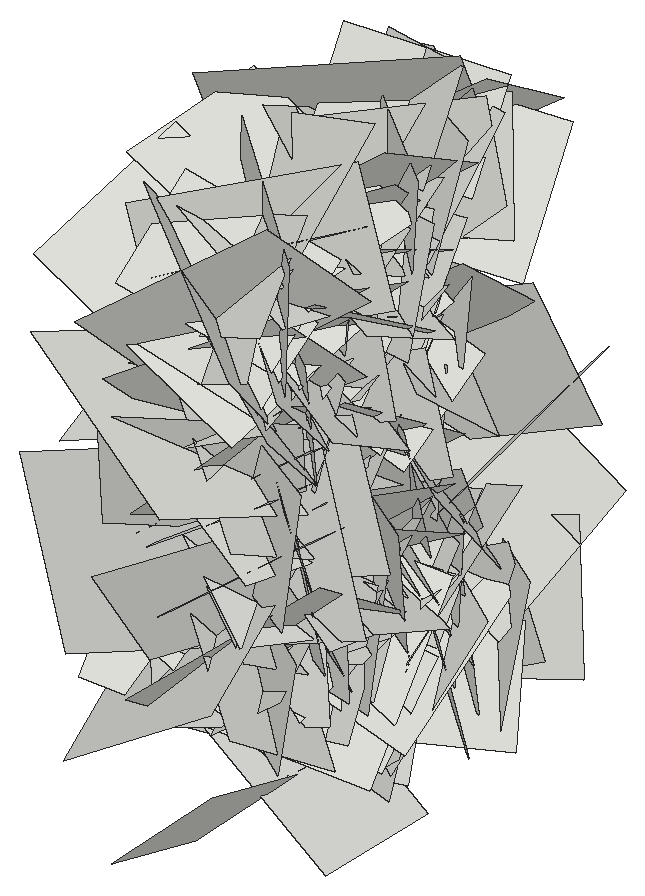
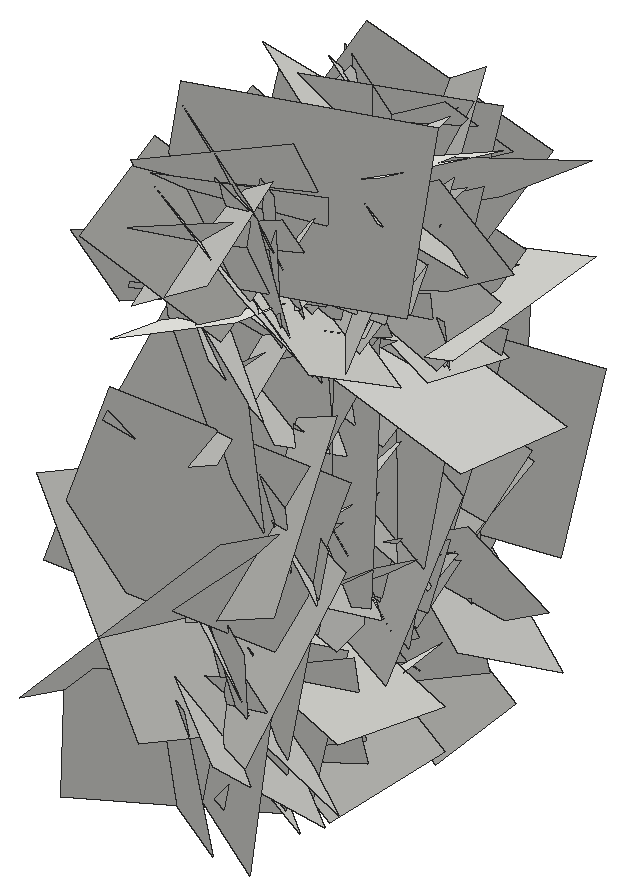
# SketchUp Ruby script. Lengths in inches.
U = 1.inch
M = Sketchup.active_model
def pt(a) = Geom::Point3d.new(a.map { |v| v * U })
def face(e, loops, mat)
  f = e.add_face(loops[0].map { |a| pt(a) })
  loops[1..].each { |l| e.add_face(l.map { |a| pt(a) }).erase! }
  f.material = f.back_material = mat if mat
  f
end
# faces: each face lists its corners as indices into pts; further lists are holes
def faces(e, pts, list, mat = nil) = list.each { |f| face(e, (f[0].is_a?(Array) ? f : [f]).map { |l| l.map { |i| pts[i] } }, mat) }
# xy, xz, yz: faces in a plane at the given z, y or x. An outline is a flat list of corners, or four numbers for a rectangle; further outlines are holes
def ring(l) = l.size == 4 ? [[l[0], l[1]], [l[2], l[1]], [l[2], l[3]], [l[0], l[3]]] : l.each_slice(2).to_a
def flat(e, list, mat, &to3) = list.each { |f| face(e, (f[0].is_a?(Array) ? f : [f]).map { |l| ring(l).map { |u, v| to3.(u, v) } }, mat) }
def xy(e, z, list, mat = nil) = flat(e, list, mat) { |x, y| [x, y, z] }
def xz(e, y, list, mat = nil) = flat(e, list, mat) { |x, z| [x, y, z] }
def yz(e, x, list, mat = nil) = flat(e, list, mat) { |y, z| [x, y, z] }
def lines(e, pts, list) = list.each { |a, b| e.add_line(pt(pts[a]), pt(pts[b])) }
# prism: a flat outline (further loops are holes) pulled along v
def prism(e, loops, v, mat = nil)
  f = face(e, loops, mat); d = Geom::Vector3d.new(v.map { |x| x * U })
  f.pushpull(f.normal.samedirection?(d) ? d.length : -d.length)
end
def box(e, o, s, mat = nil) = prism(e, [[o, [o[0] + s[0], o[1], o[2]], [o[0] + s[0], o[1] + s[1], o[2]], [o[0], o[1] + s[1], o[2]]]], [0, 0, s[2]], mat)
def at(x, y, z, deg = 0) = Geom::Transformation.translation(pt([x, y, z])) * Geom::Transformation.rotation(ORIGIN, Z_AXIS, deg.degrees)
def axes(o, x, y, z) = Geom::Transformation.new([*x, 0, *y, 0, *z, 0, *pt(o).to_a, 1])
def part(name) = M.definitions.add(name)
# library, detail: a bought-in or finely detailed component or shape, given as its bounding box
def library(name, o, s) = part(name).tap { |d| box(d.entities, o, s) }
def detail(e, o, s) = box(e.add_group.entities, o, s)
def put(e, d, t, mat = nil) = e.add_instance(d, t).tap { |i| i.material = mat if mat }
def group(e, t, mat = nil) = e.add_group.tap { |g| g.transformation = t; g.material = mat if mat }.entities
root = M.entities
c1 = part("Component\#6")
p = [[0.01,0,0],[0,3.24,4.54],[4.32,3.24,4.54],[4.33,0,0]]
faces(c1.entities,p,[[0,1,2,3]])
put(root,c1,axes([18.5,193.54,33.12],[-0.22081,1.30446,0.31828],[-0.37279,0.25784,-1.28691],[-1.3736,-0.27967,0.29809]))
put(root,c1,axes([18.5,195.625,24.52],[-0.22176,-0.47224,1.18941],[-0.10161,1.2076,0.46259],[-1.3527,-0.0133,-0.22974]))
put(root,c1,axes([18.5,200.57,23.13],[-0.2198,-0.69796,1.13548],[0.0671,1.14269,0.71395],[-1.41122,0.16304,-0.1429]))
put(root,c1,axes([18.5,199.97,41.09],[-0.2759,0.65189,-0.94787],[-0.07756,-0.97924,-0.65337],[-1.21695,-0.08538,0.25653]))
put(root,c1,axes([18.5,193.84,30.46],[-0.25587,-1.06575,0.3461],[-0.15582,0.3811,1.07099],[-1.17751,0.18115,-0.21693]))
put(root,c1,axes([18.5,194.52,25.48],[-0.11423,-0.20624,1.26777],[-0.06819,1.2715,0.20138],[-1.3598,-0.04643,-0.1166]))
put(root,c1,axes([18.5,189.88,26.35],[-0.12674,1.17916,0.69894],[0.07675,0.70605,-1.17877],[-1.45096,-0.06565,-0.1234]))
put(root,c1,axes([18.5,196.54,35.06],[-0.17609,-1.11494,-0.45613],[0.00034,-0.46049,1.12547],[-1.27691,0.15363,0.0632]))
put(root,c1,axes([18.5,199.72,26.12],[0.08735,-0.8928,-1.02237],[-0.07635,-1.02569,0.88989],[-1.43674,0.00023,-0.10945]))
put(root,c1,axes([18.5,196.35,30.1],[-0.25467,1.00338,0.64071],[0.12934,0.67094,-1.00496],[-1.25528,-0.13443,-0.23354]))
put(root,c1,axes([18.5,198.29,23.22],[-0.04433,-0.32511,1.32538],[0.126,1.3201,0.32757],[-1.44106,0.12543,-0.01213]))
put(root,c1,axes([18.5,200.75,21.625],[-0.14431,-0.01788,1.13958],[-0.06693,1.14604,0.01044],[-1.20625,-0.06145,-0.13692]))
put(root,c1,axes([18.5,197.21,31.46],[-0.04455,0.58157,-0.95839],[-0.2239,-0.94599,-0.56478],[-1.16701,0.1593,0.14494]))
put(root,c1,axes([18.5,198.24,37.08],[-0.15669,-0.99926,-0.19378],[-0.22295,-0.1616,0.99377],[-1.05566,0.18244,-0.18112]))
put(root,c1,axes([18.5,193.85,32.27],[-0.12737,1.17977,-0.33684],[0.1012,-0.32843,-1.18439],[-1.29659,-0.14153,-0.05935]))
put(root,c1,axes([18.5,196.04,25.17],[-0.02819,1.07686,0.22249],[-0.25409,0.21152,-1.05244],[-1.13755,-0.07393,0.22957]))
put(root,c1,axes([18.5,194.3,32.47],[0.23408,0.14056,-1.33491],[-0.22407,-1.33233,-0.17526],[-1.40507,0.23589,-0.19445]))
put(root,c1,axes([18.5,197.73,24.08],[-0.06299,0.80841,0.87356],[0.01823,0.87514,-0.8087],[-1.26151,-0.02772,-0.0553]))
put(root,c1,axes([18.5,195.34,33.06],[-0.01901,1.14103,-0.72029],[0.19621,-0.71146,-1.13165],[-1.41679,-0.11384,-0.14706]))
put(root,c1,axes([18.5,196.35,35.86],[-0.06555,0.97369,0.5362],[-0.0688,0.53295,-0.97527],[-1.17625,-0.08544,0.02716]))
put(root,c1,axes([18.5,198.78,35.93],[-0.06513,-0.64723,-0.92238],[-0.00055,-0.92374,0.64822],[-1.19442,0.03572,0.05]))
put(root,c1,axes([18.5,200.11,31.93],[-0.08158,0.26048,1.04137],[-0.05734,1.04178,-0.26458],[-1.13642,-0.07126,-0.06141]))
put(root,c1,axes([18.5,202.23,24.6],[0.19755,-1.2824,-0.48224],[0.04087,-0.48158,1.29554],[-1.4517,-0.18807,-0.02915]))
put(root,c1,axes([14.53,203.75,35.72],[-0.12855,-0.35471,-0.52952],[-0.05195,-0.53223,0.36775],[0.67359,-0.10874,-0.07269]))
put(root,c1,axes([18.5,192.77,37.47],[0.01566,0.85002,0.74451],[-0.07038,0.74394,-0.84805],[-1.19569,-0.03266,0.05967]))
put(root,c1,axes([18.5,197.22,25.56],[-0.17769,-0.12121,-0.94504],[-0.07151,-0.95564,0.13453],[-1.00742,0.08922,0.15714]))
put(root,c1,axes([18.5,195.04,27.27],[-0.2131,0.57774,0.71728],[-0.02179,0.73117,-0.59469],[-0.97604,-0.14247,-0.14333]))
put(root,c1,axes([18.5,201.66,25.46],[0.21728,-0.88431,0.94199],[-0.03627,0.94972,0.89901],[-1.36907,-0.16551,0.12568]))
put(root,c1,axes([18.5,202.95,33.21],[0.17447,0.42234,-1.07867],[-0.17991,-1.06896,-0.44444],[-1.21466,0.21899,-0.08911]))
put(root,c1,axes([18.5,199.05,27.98],[-0.08019,0.19915,0.92966],[-0.13728,0.92174,-0.20799],[-0.9984,-0.14274,-0.04607]))
put(root,c1,axes([18.5,197.83,24.35],[0.09568,0.96283,0.81475],[0.1112,0.80827,-0.9668],[-1.33234,0.1366,-0.02218]))
put(root,c1,axes([18.5,191.97,33.56],[-0.08688,0.89449,0.25558],[-0.12211,0.24484,-0.89383],[-0.97851,-0.10998,0.08885]))
put(root,c1,axes([18.5,196.22,30.25],[0.08073,-0.93811,0.99109],[0.27356,0.98462,0.91216],[-1.42044,0.13631,0.232]))
put(root,c1,axes([14.53,194.26,19.42],[-0.05867,-0.70774,0.13488],[-0.12622,0.14241,0.69835],[0.75321,-0.03127,0.12754]))
put(root,c1,axes([18.5,199.8,22.82],[0.00598,0.07204,1.08492],[0.02761,1.08461,-0.07215],[-1.15221,0.02636,0.0039]))
put(root,c1,axes([14.53,192.39,25.48],[-0.15082,-0.34829,0.66058],[-0.01541,0.67363,0.35204],[0.79143,-0.05326,0.13274]))
put(root,c1,axes([14.53,196.3,29.33],[-0.09147,0.43894,-0.4809],[0.05464,-0.47898,-0.44644],[0.688,0.09639,-0.02848]))
put(root,c1,axes([18.5,197.85,24.73],[0.35143,-0.52734,1.13432],[-0.18025,1.14359,0.58135],[-1.31365,-0.29799,0.22369]))
put(root,c1,axes([18.5,193.58,33.2],[-0.1306,0.22319,-0.86205],[-0.05382,-0.87061,-0.21815],[-0.94237,0.01879,0.13193]))
put(root,c1,axes([18.5,198.8,27.02],[0.0226,-0.2767,0.96977],[-0.06915,0.96758,0.27751],[-1.06674,-0.06859,0.00256]))
put(root,c1,axes([18.5,197.34,38.49],[-0.22162,0.66132,-0.53694],[0.02723,-0.54773,-0.68462],[-0.90256,-0.17891,0.1112]))
put(root,c1,axes([14.53,200.57,36.04],[-0.10099,0.61602,0.17436],[0.1325,0.19079,-0.60575],[0.66557,0.05549,0.14705]))
put(root,c1,axes([18.5,195.125,35.61],[-0.03117,0.92717,-0.40656],[0.02653,-0.40594,-0.92757],[-1.07281,-0.03698,-0.01113]))
put(root,c1,axes([14.53,198.68,37.125],[0.06347,0.58127,-0.24952],[-0.07215,-0.24326,-0.58302],[0.66662,-0.08167,-0.03935]))
put(root,c1,axes([14.53,193.25,29.42],[-0.0602,0.67546,-0.3863],[-0.10598,-0.39045,-0.66802],[0.81797,-0.00088,-0.11498]))
put(root,c1,axes([14.53,194.71,36.49],[-0.01491,0.71707,-0.22931],[-0.11795,-0.22881,-0.70868],[0.78925,-0.02064,-0.11024]))
put(root,c1,axes([18.5,198.67,35.61],[0.10111,0.59855,0.78971],[-0.15679,0.79307,-0.58323],[-1.03859,-0.06146,0.16492]))
put(root,c1,axes([18.5,206.72,25.52],[0.07134,-1.27871,-0.42932],[0.37284,-0.39835,1.24159],[-1.38032,-0.17369,0.31318]))
put(root,c1,axes([18.5,196.41,37.05],[-0.02372,0.78814,-0.36288],[-0.15491,-0.36124,-0.77556],[-0.90659,0.0411,0.14202]))
put(root,c1,axes([18.5,200.08,36.17],[-0.04967,-0.3024,-0.77978],[-0.15753,-0.76557,0.30582],[-0.87244,0.15545,-0.01082]))
put(root,c1,axes([14.53,194.0625,27.88],[-0.03826,-0.32146,0.75655],[-0.14724,0.74878,0.31153],[0.85881,0.11405,0.08712]))
put(root,c1,axes([14.53,192.62,23.41],[-0.0945,0.05137,0.75973],[0.00531,0.76494,-0.05113],[0.80713,0.00098,0.08928]))
put(root,c1,axes([14.53,194.1,30.97],[-0.07757,0.18705,0.69229],[0.05179,0.69557,-0.18277],[0.75837,-0.02837,0.08329]))
put(root,c1,axes([18.5,192.76,27.5],[0.21382,-0.08753,1.03604],[-0.20559,1.03367,0.1251],[-1.08277,-0.21355,0.18084]))
put(root,c1,axes([14.53,197.11,20.7],[-0.0234,0.20043,0.60552],[0.11848,0.59772,-0.19378],[0.66563,-0.09934,0.05578]))
put(root,c1,axes([18.5,194.12,36.42],[0.16155,0.92195,-0.51802],[-0.06641,-0.51458,-0.93426],[-1.119,0.16364,-0.01934]))
put(root,c1,axes([14.53,192.68,25.51],[0.10584,0.56729,0.32604],[-0.07365,0.33715,-0.56532],[0.68964,-0.05105,-0.11041]))
put(root,c1,axes([18.5,198.72,19.65],[0.06387,-1.04135,0.05905],[0.06023,0.06234,1.04135],[-1.10396,-0.05685,0.06023]))
put(root,c1,axes([18.5,194.92,22.54],[-0.07164,-0.895,0.57486],[0.24411,0.55005,0.88344],[-1.1008,0.18023,0.15849]))
put(root,c1,axes([18.5,200.17,25.9],[-0.12286,-0.34825,-0.84521],[0.12526,-0.85054,0.33424],[-0.96086,-0.06635,0.15165]))
put(root,c1,axes([14.53,196.5,26.6],[-0.00001,0.64808,0.59207],[-0.20568,0.57742,-0.63205],[0.90746,0.13088,-0.14325]))
put(root,c1,axes([18.5,195.45,23.05],[-0.08121,0.42866,0.62692],[-0.16296,0.6083,-0.43472],[-0.78836,-0.1699,0.02528]))
put(root,c1,axes([14.53,201.07,39.9375],[-0.03161,0.68058,-0.41337],[-0.06223,-0.41441,-0.67806],[0.84176,-0.00508,-0.06565]))
put(root,c1,axes([14.53,199.74,34.07],[0.11183,-0.60219,-0.2199],[-0.02555,-0.22643,0.6085],[0.67907,0.09065,0.0591]))
put(root,c1,axes([18.5,195.7,29.31],[0.12944,0.87645,-0.3909],[-0.13192,-0.37627,-0.88251],[-1.00866,0.16168,0.06525]))
put(root,c1,axes([18.5,195.4,26.27],[-0.15303,-0.80886,0.21466],[0.08059,0.20425,0.82078],[-0.8834,0.15875,0.0377]))
put(root,c1,axes([14.53,197.17,21.41],[-0.31691,0.51794,0.91951],[-0.05422,0.94746,-0.55031],[1.11735,0.19287,0.23409]))
put(root,c1,axes([18.5,204.82,25.65],[0.12938,-0.11687,-1.00907],[-0.02351,-1.01639,0.11504],[-1.07651,0.00815,-0.12379]))
put(root,c1,axes([14.53,192.15,39.48],[-0.21361,0.71392,-0.72381],[-0.12034,-0.74908,-0.70723],[1.07091,0.05823,-0.22384]))
put(root,c1,axes([18.5,200.1,34.99],[-0.01875,0.74709,-0.59948],[0.09315,-0.59579,-0.74508],[-1.01106,-0.06874,-0.05753]))
put(root,c1,axes([14.53,198.57,33.25],[-0.09717,0.14422,-0.89801],[-0.11089,-0.89824,-0.13357],[0.95769,-0.08937,-0.10658]))
put(root,c1,axes([18.5,201.91,26.14],[0.02369,0.31708,-0.9382],[0.09459,-0.93526,-0.31396],[-1.04548,-0.07743,-0.04967]))
put(root,c1,axes([18.5,195.16,37.28],[-0.08536,-0.54597,-0.55526],[-0.06407,-0.55215,0.55168],[-0.82294,0.09962,0.01464]))
put(root,c1,axes([14.53,196.95,39.61],[-0.06663,0.78722,-0.39485],[-0.0883,-0.3994,-0.78302],[0.92935,0.01849,-0.10271]))
put(root,c1,axes([14.53,194.17,31.15],[-0.1572,-0.65225,0.62778],[-0.00257,0.63643,0.66066],[0.9596,-0.10514,0.10461]))
put(root,c1,axes([18.5,197.53,26.62],[-0.11622,-0.11144,-0.6986],[-0.08861,-0.69994,0.12478],[-0.74462,0.10068,0.09418]))
put(root,c1,axes([18.5,195.33,34.42],[-0.12228,0.30682,0.85432],[0.19875,0.85067,-0.2802],[-0.94146,0.13973,-0.17012]))
put(root,c1,axes([14.53,195.89,35.57],[-0.03273,-0.74668,0.19464],[0.06894,0.19158,0.74527],[0.81502,-0.04619,-0.05522]))
put(root,c1,axes([14.53,192.38,31.46],[0.05244,0.73173,-0.11131],[0.01157,-0.11227,-0.73318],[0.78447,-0.04726,0.01825]))
put(root,c1,axes([18.5,198.41,25.5],[0.14641,-1.02966,0.26735],[0.10928,0.28128,1.03005],[-1.12233,-0.10694,0.13517]))
put(root,c1,axes([18.5,198.86,35.2],[0.14047,0.16017,0.87964],[-0.13868,0.88315,-0.1411],[-0.93754,-0.10664,0.15267]))
put(root,c1,axes([14.53,193.07,33.95],[0.05953,0.85388,-0.40475],[-0.24794,-0.38029,-0.83472],[0.97048,-0.14953,-0.18843]))
put(root,c1,axes([14.53,201.02,39.48],[-0.13577,0.09163,-0.9618],[-0.05798,-0.96935,-0.08506],[1.02248,-0.0428,-0.13253]))
put(root,c1,axes([14.53,192.92,34.17],[-0.15147,-0.1521,1.01718],[-0.1212,1.02293,0.1369],[1.08344,0.09316,0.15752]))
put(root,c1,axes([18.5,191.375,35.34],[-0.1473,0.40574,0.51918],[-0.07991,0.51733,-0.42447],[-0.69387,-0.14571,-0.06134]))
put(root,c1,axes([18.5,194.18,31.13],[0.04063,-0.16003,0.87853],[0.02386,0.87924,0.15917],[-0.94627,0.0153,0.04174]))
put(root,c1,axes([14.53,202.06,39.63],[-0.00244,-0.36914,-0.6705],[0.07457,-0.66776,0.36739],[0.80789,0.06052,-0.03594]))
put(root,c1,axes([18.5,201.02,32],[0.03236,-0.79816,-0.43551],[0.07074,-0.43262,0.79753],[-0.9612,-0.0587,0.04403]))
put(root,c1,axes([18.5,199.18,25.47],[-0.11604,-0.3767,0.6399],[0.02749,0.64448,0.38383],[-0.78661,0.07809,-0.08099]))
put(root,c1,axes([14.53,199.18,25.47],[0.11604,-0.3767,0.6399],[-0.02749,0.64448,0.38383],[0.78661,0.07809,-0.08099]))
put(root,c1,axes([14.53,201.02,32],[-0.03236,-0.79816,-0.43551],[-0.07074,-0.43262,0.79753],[0.9612,-0.0587,0.04403]))
put(root,c1,axes([18.5,202.06,39.63],[0.00244,-0.36914,-0.6705],[-0.07457,-0.66776,0.36739],[-0.80789,0.06052,-0.03594]))
put(root,c1,axes([14.53,194.18,31.13],[-0.04063,-0.16003,0.87853],[-0.02386,0.87924,0.15917],[0.94627,0.0153,0.04174]))
put(root,c1,axes([14.53,191.375,35.34],[0.1473,0.40574,0.51918],[0.07991,0.51733,-0.42447],[0.69387,-0.14571,-0.06134]))
put(root,c1,axes([18.5,192.92,34.17],[0.15147,-0.1521,1.01718],[0.1212,1.02293,0.1369],[-1.08344,0.09316,0.15752]))
put(root,c1,axes([18.5,201.02,39.48],[0.13577,0.09163,-0.9618],[0.05798,-0.96935,-0.08506],[-1.02248,-0.0428,-0.13253]))
put(root,c1,axes([18.5,193.07,33.95],[-0.05953,0.85388,-0.40475],[0.24794,-0.38029,-0.83472],[-0.97048,-0.14953,-0.18843]))
put(root,c1,axes([14.53,198.86,35.2],[-0.14047,0.16017,0.87964],[0.13868,0.88315,-0.1411],[0.93754,-0.10664,0.15267]))
put(root,c1,axes([14.53,198.41,25.5],[-0.14641,-1.02966,0.26735],[-0.10928,0.28128,1.03005],[1.12233,-0.10694,0.13517]))
put(root,c1,axes([18.5,192.38,31.46],[-0.05244,0.73173,-0.11131],[-0.01157,-0.11227,-0.73318],[-0.78447,-0.04726,0.01825]))
put(root,c1,axes([18.5,195.89,35.57],[0.03273,-0.74668,0.19464],[-0.06894,0.19158,0.74527],[-0.81502,-0.04619,-0.05522]))
put(root,c1,axes([14.53,195.33,34.42],[0.12228,0.30682,0.85432],[-0.19875,0.85067,-0.2802],[0.94146,0.13973,-0.17012]))
put(root,c1,axes([14.53,197.53,26.62],[0.11622,-0.11144,-0.6986],[0.08861,-0.69994,0.12478],[0.74462,0.10068,0.09418]))
put(root,c1,axes([18.5,194.17,31.15],[0.1572,-0.65225,0.62778],[0.00257,0.63643,0.66066],[-0.9596,-0.10514,0.10461]))
put(root,c1,axes([18.5,196.95,39.61],[0.06663,0.78722,-0.39485],[0.0883,-0.3994,-0.78302],[-0.92935,0.01849,-0.10271]))
put(root,c1,axes([14.53,195.16,37.28],[0.08536,-0.54597,-0.55526],[0.06407,-0.55215,0.55168],[0.82294,0.09962,0.01464]))
put(root,c1,axes([14.53,201.91,26.14],[-0.02369,0.31708,-0.9382],[-0.09459,-0.93526,-0.31396],[1.04548,-0.07743,-0.04967]))
put(root,c1,axes([18.5,198.57,33.25],[0.09717,0.14422,-0.89801],[0.11089,-0.89824,-0.13357],[-0.95769,-0.08937,-0.10658]))
put(root,c1,axes([14.53,200.1,34.99],[0.01875,0.74709,-0.59948],[-0.09315,-0.59579,-0.74508],[1.01106,-0.06874,-0.05753]))
put(root,c1,axes([18.5,192.15,39.48],[0.21361,0.71392,-0.72381],[0.12034,-0.74908,-0.70723],[-1.07091,0.05823,-0.22384]))
put(root,c1,axes([14.53,204.82,25.65],[-0.12938,-0.11687,-1.00907],[0.02351,-1.01639,0.11504],[1.07651,0.00815,-0.12379]))
put(root,c1,axes([18.5,197.17,21.41],[0.31691,0.51794,0.91951],[0.05422,0.94746,-0.55031],[-1.11735,0.19287,0.23409]))
put(root,c1,axes([14.53,195.4,26.27],[0.15303,-0.80886,0.21466],[-0.08059,0.20425,0.82078],[0.8834,0.15875,0.0377]))
put(root,c1,axes([14.53,195.7,29.31],[-0.12944,0.87645,-0.3909],[0.13192,-0.37627,-0.88251],[1.00866,0.16168,0.06525]))
put(root,c1,axes([18.5,199.74,34.07],[-0.11183,-0.60219,-0.2199],[0.02555,-0.22643,0.6085],[-0.67907,0.09065,0.0591]))
put(root,c1,axes([18.5,201.07,39.9375],[0.03161,0.68058,-0.41337],[0.06223,-0.41441,-0.67806],[-0.84176,-0.00508,-0.06565]))
put(root,c1,axes([14.53,195.45,23.05],[0.08121,0.42866,0.62692],[0.16296,0.6083,-0.43472],[0.78836,-0.1699,0.02528]))
put(root,c1,axes([18.5,196.5,26.6],[0.00001,0.64808,0.59207],[0.20568,0.57742,-0.63205],[-0.90746,0.13088,-0.14325]))
put(root,c1,axes([14.53,200.17,25.9],[0.12286,-0.34825,-0.84521],[-0.12526,-0.85054,0.33424],[0.96086,-0.06635,0.15165]))
put(root,c1,axes([14.53,194.92,22.54],[0.07164,-0.895,0.57486],[-0.24411,0.55005,0.88344],[1.1008,0.18023,0.15849]))
put(root,c1,axes([14.53,198.72,19.65],[-0.06387,-1.04135,0.05905],[-0.06023,0.06234,1.04135],[1.10396,-0.05685,0.06023]))
put(root,c1,axes([18.5,192.68,25.51],[-0.10584,0.56729,0.32604],[0.07365,0.33715,-0.56532],[-0.68964,-0.05105,-0.11041]))
put(root,c1,axes([14.53,194.12,36.42],[-0.16155,0.92195,-0.51802],[0.06641,-0.51458,-0.93426],[1.119,0.16364,-0.01934]))
put(root,c1,axes([18.5,197.11,20.7],[0.0234,0.20043,0.60552],[-0.11848,0.59772,-0.19378],[-0.66563,-0.09934,0.05578]))
put(root,c1,axes([14.53,192.76,27.5],[-0.21382,-0.08753,1.03604],[0.20559,1.03367,0.1251],[1.08277,-0.21355,0.18084]))
put(root,c1,axes([18.5,194.1,30.97],[0.07757,0.18705,0.69229],[-0.05179,0.69557,-0.18277],[-0.75837,-0.02837,0.08329]))
put(root,c1,axes([18.5,192.62,23.41],[0.0945,0.05137,0.75973],[-0.00531,0.76494,-0.05113],[-0.80713,0.00098,0.08928]))
put(root,c1,axes([18.5,194.0625,27.88],[0.03826,-0.32146,0.75655],[0.14724,0.74878,0.31153],[-0.85881,0.11405,0.08712]))
put(root,c1,axes([14.53,200.08,36.17],[0.04967,-0.3024,-0.77978],[0.15753,-0.76557,0.30582],[0.87244,0.15545,-0.01082]))
put(root,c1,axes([14.53,196.41,37.05],[0.02372,0.78814,-0.36288],[0.15491,-0.36124,-0.77556],[0.90659,0.0411,0.14202]))
put(root,c1,axes([14.53,206.72,25.52],[-0.07134,-1.27871,-0.42932],[-0.37284,-0.39835,1.24159],[1.38032,-0.17369,0.31318]))
put(root,c1,axes([14.53,198.67,35.61],[-0.10111,0.59855,0.78971],[0.15679,0.79307,-0.58323],[1.03859,-0.06146,0.16492]))
put(root,c1,axes([18.5,194.71,36.49],[0.01491,0.71707,-0.22931],[0.11795,-0.22881,-0.70868],[-0.78925,-0.02064,-0.11024]))
